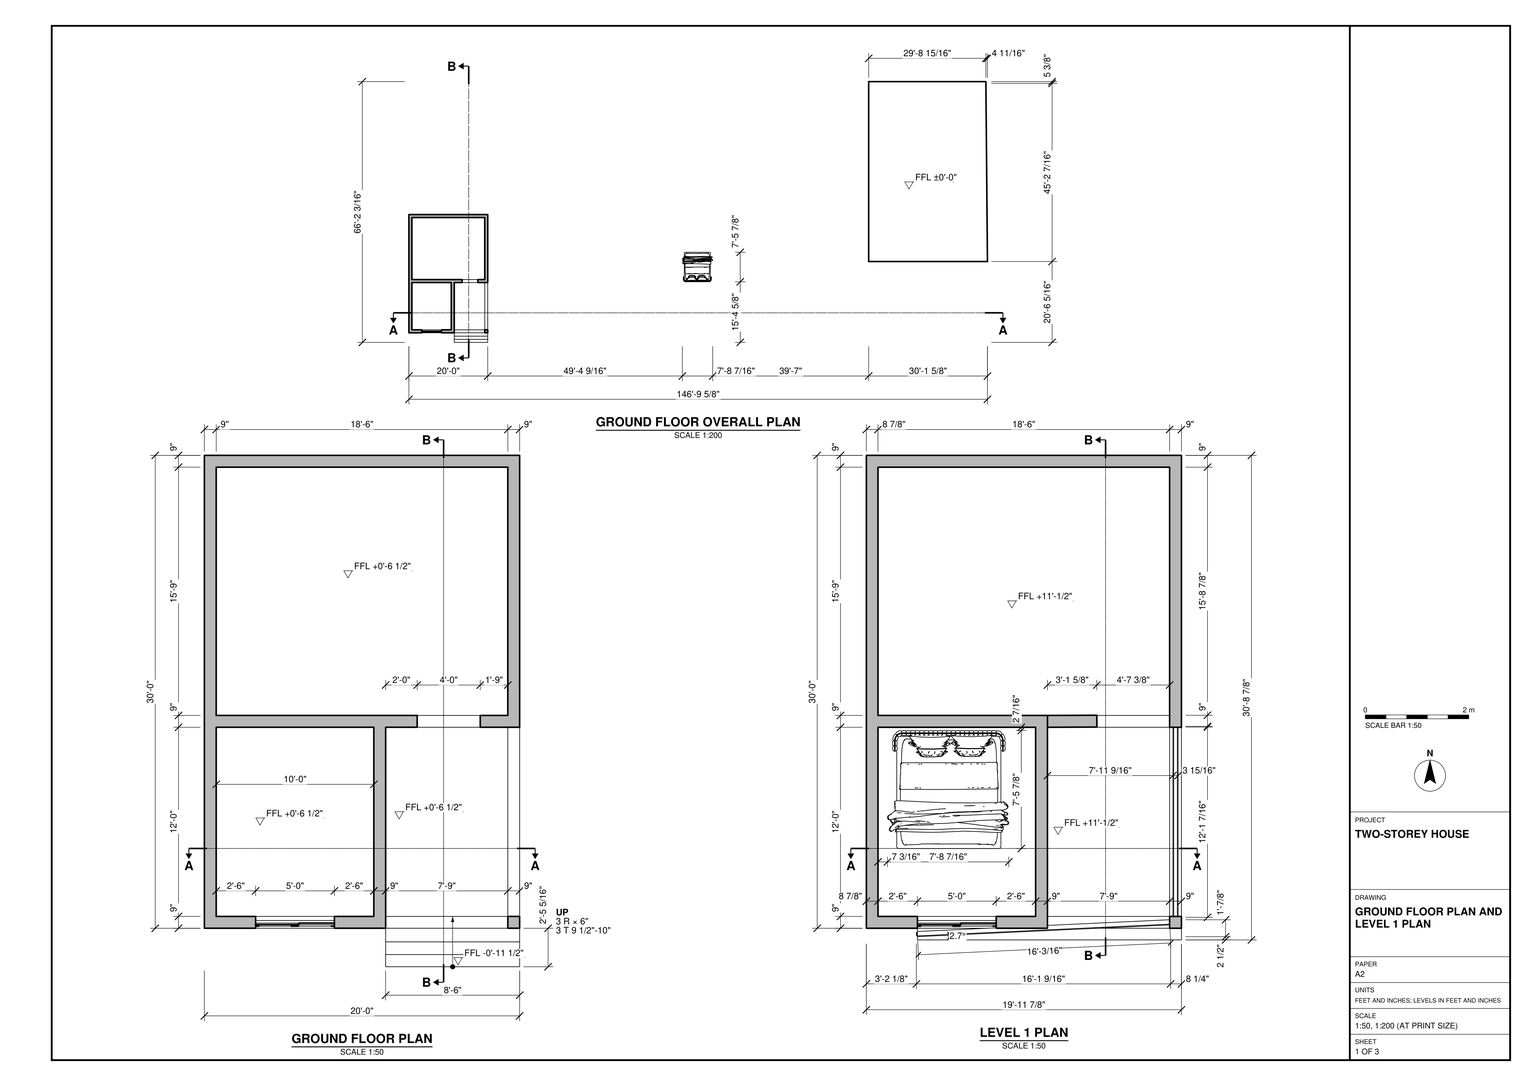
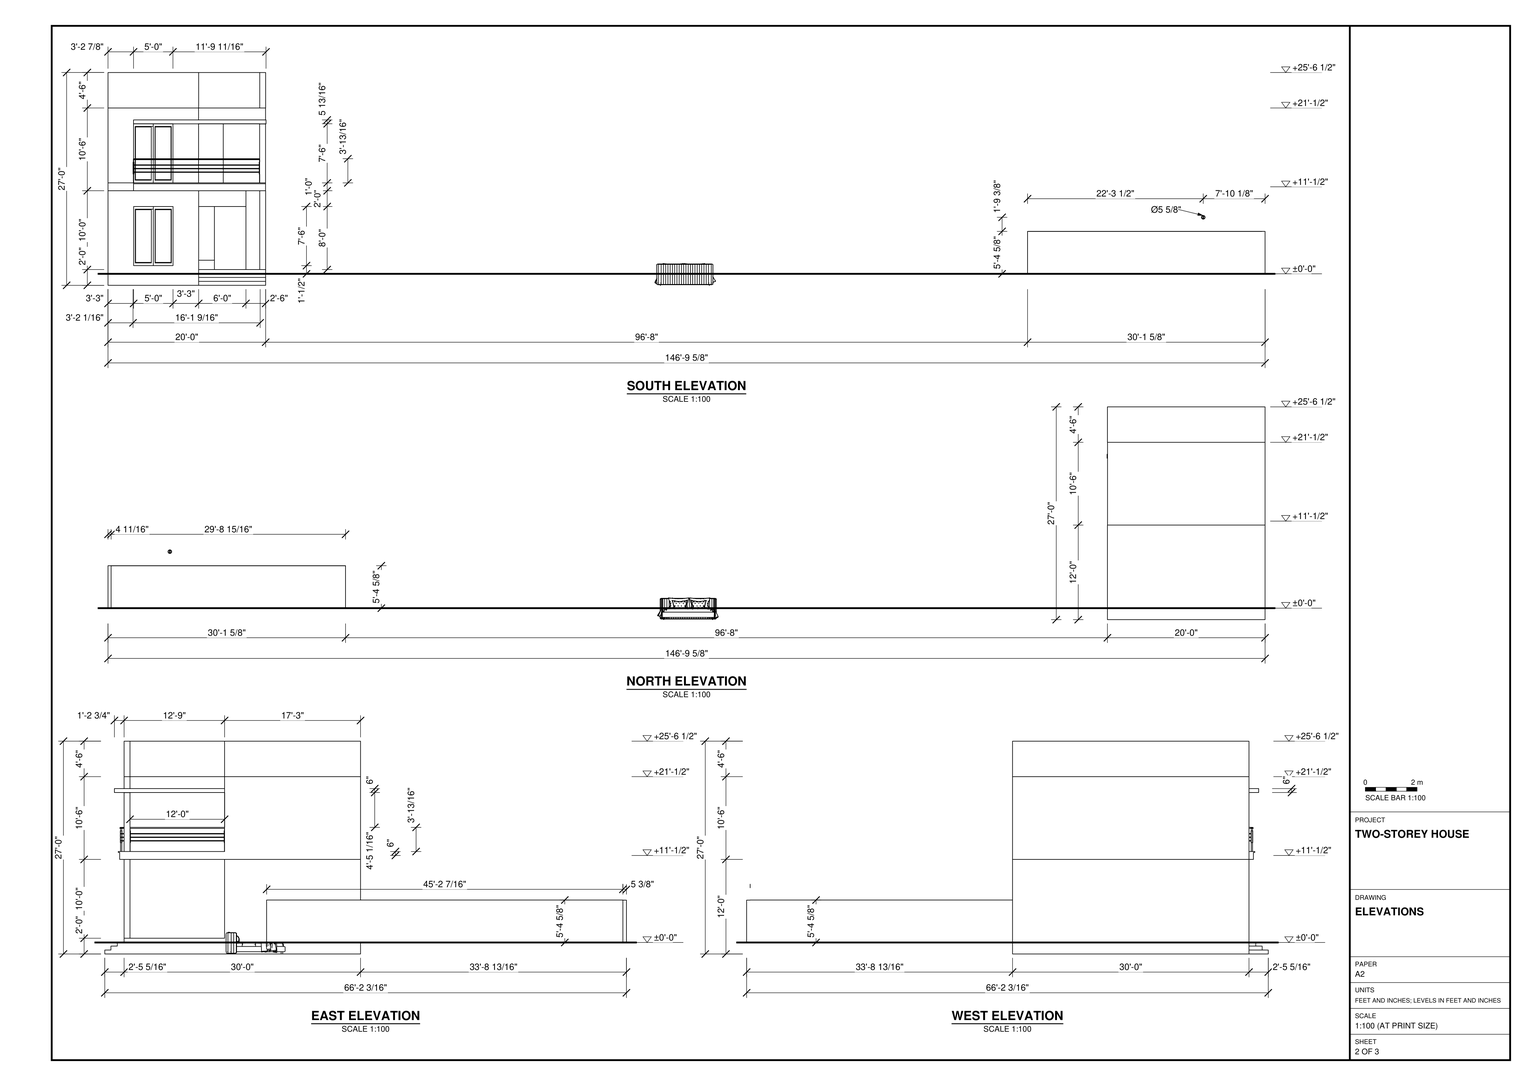
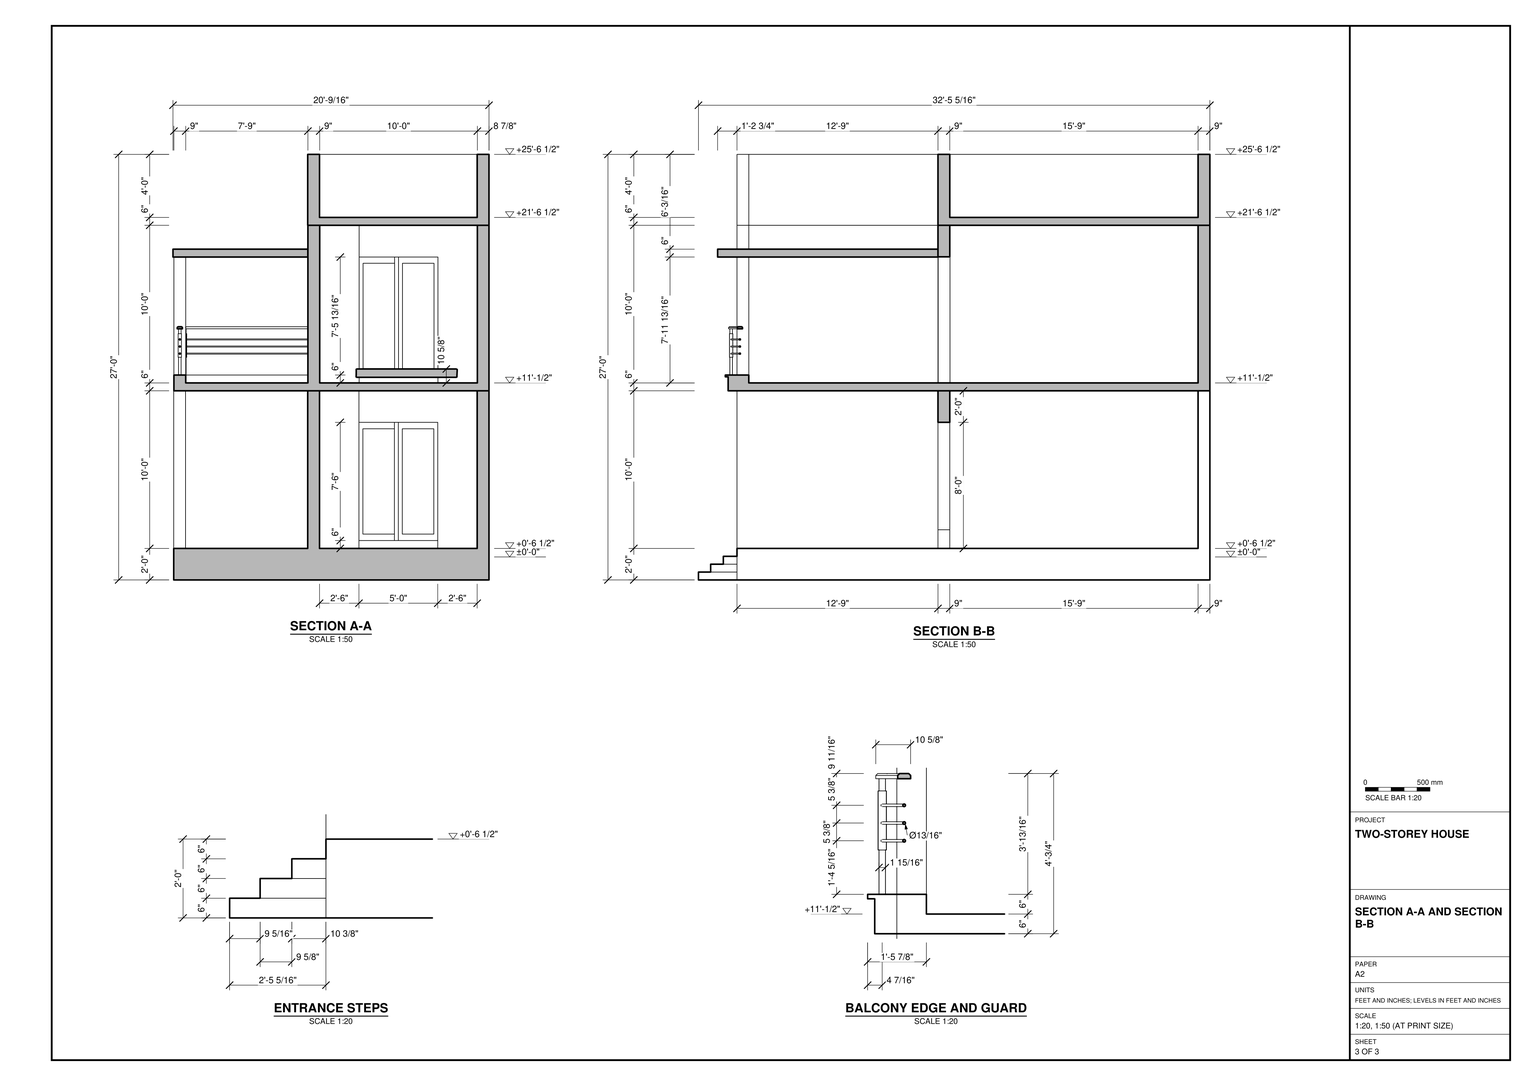
Build the house and the separate elements shown in task_files/diagram_01.pdf. Work in feet and inches. Use the overall plan to set out the full model: it measures 146'-9 5/8" east to west, 66'-2 3/16" north to south and 27'-0" high. Use ±0'-0" as the ground datum and +11'-1/2" as the upper floor level. The finished ground floor of the house sits above the datum at +0'-6 1/2".

Set out the 20'-0" by 30'-0" house at the west end. On each floor, form the full-width rear room and the smaller enclosed room at the front left, using the wall thicknesses shown in plan. Model the raised base, entrance steps, recessed entry bay, wall openings and framed window units. Follow the sections for the floor slabs, flat roof, parapets and lower canopy over the balcony. Include the balcony edge and horizontal guard rails. Place the bed in the upper front-left room as drawn. Use the overall plan and elevations to position the separate bed and the low rectangular element east of the house; they are not part of the house footprint.

Keep walls, slabs, roof elements and each furniture or joinery piece in separate groups or components, and use components for repeated parts. Decor and loose items may be any suitable library components. Save one SketchUp model as output_files/two_storey_house_with_a_covered_balcony.skp.

# SketchUp Ruby script. Lengths in inches.
U = 1.inch
M = Sketchup.active_model
def pt(a) = Geom::Point3d.new(a.map { |v| v * U })
def face(e, loops, mat)
  f = e.add_face(loops[0].map { |a| pt(a) })
  loops[1..].each { |l| e.add_face(l.map { |a| pt(a) }).erase! }
  f.material = f.back_material = mat if mat
  f
end
# faces: each face lists its corners as indices into pts; further lists are holes
def faces(e, pts, list, mat = nil) = list.each { |f| face(e, (f[0].is_a?(Array) ? f : [f]).map { |l| l.map { |i| pts[i] } }, mat) }
# xy, xz, yz: faces in a plane at the given z, y or x. An outline is a flat list of corners, or four numbers for a rectangle; further outlines are holes
def ring(l) = l.size == 4 ? [[l[0], l[1]], [l[2], l[1]], [l[2], l[3]], [l[0], l[3]]] : l.each_slice(2).to_a
def flat(e, list, mat, &to3) = list.each { |f| face(e, (f[0].is_a?(Array) ? f : [f]).map { |l| ring(l).map { |u, v| to3.(u, v) } }, mat) }
def xy(e, z, list, mat = nil) = flat(e, list, mat) { |x, y| [x, y, z] }
def xz(e, y, list, mat = nil) = flat(e, list, mat) { |x, z| [x, y, z] }
def yz(e, x, list, mat = nil) = flat(e, list, mat) { |y, z| [x, y, z] }
def lines(e, pts, list) = list.each { |a, b| e.add_line(pt(pts[a]), pt(pts[b])) }
# prism: a flat outline (further loops are holes) pulled along v
def prism(e, loops, v, mat = nil)
  f = face(e, loops, mat); d = Geom::Vector3d.new(v.map { |x| x * U })
  f.pushpull(f.normal.samedirection?(d) ? d.length : -d.length)
end
def box(e, o, s, mat = nil) = prism(e, [[o, [o[0] + s[0], o[1], o[2]], [o[0] + s[0], o[1] + s[1], o[2]], [o[0], o[1] + s[1], o[2]]]], [0, 0, s[2]], mat)
def at(x, y, z, deg = 0) = Geom::Transformation.translation(pt([x, y, z])) * Geom::Transformation.rotation(ORIGIN, Z_AXIS, deg.degrees)
def axes(o, x, y, z) = Geom::Transformation.new([*x, 0, *y, 0, *z, 0, *pt(o).to_a, 1])
def part(name) = M.definitions.add(name)
# library, detail: a bought-in or finely detailed component or shape, given as its bounding box
def library(name, o, s) = part(name).tap { |d| box(d.entities, o, s) }
def detail(e, o, s) = box(e.add_group.entities, o, s)
def put(e, d, t, mat = nil) = e.add_instance(d, t).tap { |i| i.material = mat if mat }
def group(e, t, mat = nil) = e.add_group.tap { |g| g.transformation = t; g.material = mat if mat }.entities
root = M.entities
M.materials.add("[Brick Antique 01]").color = [147, 105, 71]
M.materials.add("[Carrera Marble]").color = [207, 207, 207]
M.materials.add("[Color M05]").color = [114, 114, 114]
M.materials.add("[Color M08]").color = [30, 30, 30]
M.materials.add("[Color M09]").color = [0, 0, 0]
M.materials.add("[Translucent Glass Blue]").color = [100, 149, 237]
M.materials["[Translucent Glass Blue]"].alpha = 0.5
M.materials.add("[Wood Veneer 02]").color = [190, 128, 91]
c1 = part("Janela aluminio")
xy(c1.entities,0,[[0,0,47.24,1.57],[23.62,1.57,47.24,2.76],[0,2.76,25.98,3.9375],[0,3.9375,47.24,5.91]])
xy(c1.entities,43.31,[[0,0,47.24,1.57],[23.62,1.57,47.24,2.76],[0,2.76,0,5.91,47.24,5.91,47.24,3.9375,25.98,3.9375,25.98,2.76],[25.98,2.76,47.24,3.9375]])
xz(c1.entities,1.57,[[0,0,23.62,0,23.62,41.34,21.26,41.34,21.26,1.97,1.97,1.97,1.97,41.34,23.62,41.34,23.62,43.31,0,43.31],[[23.62,0,47.24,43.31],[25.7,1.97,45.28,41.34]]])
xz(c1.entities,2.76,[[[0,0,23.62,43.31],[2.36,2.36,21.26,40.94]],[23.62,0,25.98,43.31]])
xz(c1.entities,2.76,[[2.36,2.36,21.26,40.94]],"[Translucent Glass Blue]")
xz(c1.entities,3.9375,[[25.98,0,25.98,2.36,44.88,2.36,44.88,40.94,25.98,40.94,25.98,43.31,47.24,43.31,47.24,0]])
xz(c1.entities,3.9375,[[25.98,2.36,44.88,40.94]],"[Translucent Glass Blue]")
yz(c1.entities,0,[[0,0,1.57,43.31],[2.76,0,5.91,43.31]])
yz(c1.entities,23.62,[[1.57,0,2.76,43.31]])
yz(c1.entities,25.98,[[2.76,0,3.9375,43.31]])
yz(c1.entities,47.24,[[0,0,1.57,43.31],[1.57,0,2.76,43.31],[3.9375,0,5.91,43.31]])
c2 = library("Untitled",[0,-1.15,0],[92.42,91.04,33.3])
c3 = part("Ploe")
prism(c3.entities,[[[657.2,82.55,156],[657.29,80.58,156],[656.82,80.5625,156],[656.72,82.53,156]]],[0,0,36])
prism(c3.entities,[[[656.71,82.8,169.5],[656.83,80.29,169.5],[656.36,80.26,169.5],[656.24,82.78,169.5]]],[0,0,18],"[Wood Veneer 02]")
prism(c3.entities,[[[657.3,80.31,169.5],[657.18,82.83,169.5],[657.66,82.85,169.5],[657.77,80.33,169.5]]],[0,0,18],"[Wood Veneer 02]")
c4 = part("Group52\#1")
put(c4.entities,c3,at(0,0,0))
put(c4.entities,c3,at(1122.01,154.17,0,-180))
c5 = part("Ploe\#1")
box(c5.entities,[660.52,85.82,156],[1.97,0.47,36])
box(c5.entities,[660.25,86.29,169.5],[2.52,0.47,18],"[Wood Veneer 02]")
box(c5.entities,[660.25,85.35,169.5],[2.52,0.47,18],"[Wood Veneer 02]")
c6 = part("Group56\#1")
put(c6.entities,c5,at(0,0,0))
put(c6.entities,c5,at(1323.01,316.11,0,-180))
box(root,[231,29.33,24],[9,9,120])
p = [[39,38.33,24],[39,29.33,24],[99,38.33,24],[99,29.33,24],[162,182.33,24],[162,191.33,24],
  [210,182.33,24],[210,191.33,24]]
lines(root,p,[[0,1],[2,3],[4,5],[6,7]])
g1 = group(root,at(0,29.33,0))
box(g1,[230.86,0,156],[9,9,89.6875],"[Color M09]")
xy(g1,0,[[138,-29.33,138,0,0,0,0,360,240,360,240,-29.33]])
xy(g1,6,[[138,-29.33,240,-20.04]])
xy(g1,12,[[138,-20.04,240,-10.39]])
xy(g1,17.51,[[1400,217,1761.62,217,1756.91,759.46,1756.91,764.84,1400,764.84]])
xy(g1,18,[[138,-10.39,240,0]],"[Carrera Marble]")
xy(g1,24,[[9,9,129,153]])
xy(g1,24,[[138,0,231,9],[231,0,240,153],[138,9,231,153],[162,153,210,162],[9,162,231,351]],"[Carrera Marble]")
xy(g1,30,[[39,0,99,9]])
xy(g1,82.01,[[1400,759.46,1756.91,764.84]])
xy(g1,120,[[39,0,99,9],[162,153,210,162]])
xy(g1,144,[[0,0,138,0,138,153,210,153,210,162,9,162,9,153,129,153,129,9,9,9,9,351,231,351,231,153,240,153,240,360,0,360],[210,153,231,162]])
xy(g1,150,[[137.89,153,137.86,162,175.45,162.16,175.49,153.16]])
xy(g1,245.83,[[137.89,153,175.49,153.16,175.45,162.16,137.86,162]])
xy(g1,245.83,[[38.86,-14.75,38.86,0,137.89,0,137.89,153,240.5625,153,240.5625,-14.75]],"[Carrera Marble]")
xy(g1,251.83,[[38.86,-14.75,240.5625,-14.75,240.5625,153,137.89,153,137.89,0,38.86,0]],"[Carrera Marble]")
xy(g1,270,[[0,0,0,360,240,360,240,153,138,153,138,0]],"[Brick Antique 01]")
xy(g1,276,[[9,9,129,9,129,162,231,162,231,351,9,351]],"[Brick Antique 01]")
xy(g1,324,[[[0,0,138,0,138,153,240,153,240,360,0,360],[9,9,9,351,231,351,231,162,129,162,129,9]]],"[Brick Antique 01]")
xz(g1,-29.33,[[138,0,240,6]],"[Carrera Marble]")
xz(g1,-20.04,[[138,6,240,12]],"[Carrera Marble]")
xz(g1,-14.75,[[38.86,245.83,240.5625,251.83]],"[Carrera Marble]")
xz(g1,-10.39,[[138,12,240,18]],"[Carrera Marble]")
xz(g1,0,[[38.86,245.83,137.89,251.83]])
xz(g1,0,[[[0,0,138,144],[39,30,99,120]],[0,270,138,324]],"[Brick Antique 01]")
xz(g1,0,[[138,18,240,24],[231,24,240,144]],"[Carrera Marble]")
xz(g1,9,[[9,24,9,144,99,144,99,120,39,120,39,24],[39,24,99,30],[99,24,129,144]])
xz(g1,9,[[9,276,129,324]],"[Brick Antique 01]")
xz(g1,153,[[9,24,129,144],[137.89,245.83,240.5625,251.83]])
xz(g1,153,[[138,24,162,38.2],[210,24,231,144],[231,24,240,144],[138,38.2,162,120],[138,120,210,144],
  [138,270,231,324],[231,270,240,324]],"[Brick Antique 01]")
xz(g1,162,[[9,24,9,144,210,144,210,120,162,120,162,38.2,138,38.2,138,24],[138,24,162,38.2],[210,24,231,144]])
xz(g1,162,[[129,276,231,324]],"[Brick Antique 01]")
xz(g1,217,[[1400,17.51,1761.62,82.15]])
xz(g1,351,[[9,276,231,324]],"[Brick Antique 01]")
xz(g1,351,[[9,24,231,144]],"[Carrera Marble]")
xz(g1,360,[[0,0,240,144]])
xz(g1,360,[[0,270,240,324]],"[Brick Antique 01]")
xz(g1,759.46,[[1667.49,100.73,1667.58,100.74,1667.49,103.54,1667.39,100.74],[[1667.39,100.74,1667.49,103.54,1667.39,106.33,1666.76,106.25,1666.08,105.97,1665.5,105.52,1665.05,104.94,1664.77,104.26,1664.68,103.54,1664.77,102.81,1665.05,102.13,1665.5,101.55,1666.08,101.1,1666.76,100.82],[1666.96,101.24,1666.88,101.26,1666.31,101.49,1665.82,101.87,1665.44,102.36,1665.21,102.93,1665.13,103.54,1665.21,104.15,1665.44,104.72,1665.82,105.21,1666.31,105.58,1666.88,105.82,1666.96,105.83,1667.04,103.54]],[[1667.58,100.74,1668.22,100.82,1668.89,101.1,1669.48,101.55,1669.92,102.13,1670.2,102.81,1670.3,103.54,1670.2,104.26,1669.92,104.94,1669.48,105.52,1668.89,105.97,1668.22,106.25,1667.58,106.33,1667.49,103.54],[1668,101.23,1667.92,103.54,1668,105.84,1668.1,105.83,1668.67,105.59,1669.17,105.21,1669.54,104.72,1669.78,104.15,1669.86,103.54,1669.78,102.92,1669.54,102.35,1669.17,101.86,1668.67,101.48,1668.1,101.24]],[1668,101.23,1668.1,101.24,1668.67,101.48,1669.17,101.86,1669.54,102.35,1669.78,102.92,1669.86,103.54,1669.78,104.15,1669.54,104.72,1669.17,105.21,1668.67,105.59,1668.1,105.83,1668,105.84,1667.92,103.54],[1666.96,101.24,1667.04,103.54,1666.96,105.83,1666.88,105.82,1666.31,105.58,1665.82,105.21,1665.44,104.72,1665.21,104.15,1665.13,103.54,1665.21,102.93,1665.44,102.36,1665.82,101.87,1666.31,101.49,1666.88,101.26],
  [1667.49,103.54,1667.58,106.33,1667.49,106.35,1667.39,106.33]])
xz(g1,764.84,[[1400,17.51,1756.91,82.01]])
yz(g1,0,[[0,0,360,144],[0,270,360,324]],"[Brick Antique 01]")
yz(g1,9,[[9,24,153,144],[162,24,351,144]])
yz(g1,9,[[9,276,351,324]],"[Brick Antique 01]")
yz(g1,38.86,[[-14.75,245.83,0,251.83]])
yz(g1,39,[[0,30,9,120]])
yz(g1,99,[[0,30,9,120]])
yz(g1,129,[[9,24,153,144]])
yz(g1,129,[[9,276,162,324]],"[Brick Antique 01]")
yz(g1,137.89,[[0,245.83,153,251.83]])
yz(g1,138,[[0,24,153,144],[0,270,9,324],[9,270,153,324]],"[Brick Antique 01]")
yz(g1,138,[[-29.33,0,0,6],[-20.04,6,0,12],[-10.39,12,0,18]],"[Carrera Marble]")
yz(g1,162,[[153,24,162,38.2],[153,38.2,162,120]],"[Brick Antique 01]")
yz(g1,210,[[153,24,162,120]])
yz(g1,231,[[162,24,351,144]])
yz(g1,231,[[162,276,351,324]],"[Brick Antique 01]")
yz(g1,231,[[0,24,9,144]],"[Color M09]")
yz(g1,240,[[-29.33,0,360,0,360,144,153,144,153,24,0,24,0,18,-10.39,18,-10.39,12,-20.04,12,-20.04,6,-29.33,6],[153,270,360,324]],"[Brick Antique 01]")
yz(g1,240,[[0,24,9,144]],"[Color M08]")
yz(g1,240.5625,[[-14.75,245.83,153,251.83]],"[Carrera Marble]")
yz(g1,1400,[[217,17.51,764.84,17.51,764.84,82.01,759.46,82.01,759.46,82.15,217,82.15]])
yz(g1,1756.91,[[759.46,17.51,764.84,82.01]])
p = [[1761.62,217,17.51],[1761.62,217,82.15],[1756.91,759.46,82.15],[1756.91,759.46,82.01],[1756.91,759.46,17.51],[137.89,153,245.83],
  [137.86,162,245.83],[137.86,162,150],[137.89,153,150],[175.49,153.16,150],[175.49,153.16,245.83],[175.45,162.16,245.83],
  [175.45,162.16,150]]
faces(g1,p,[[0,1,2,3,4],[5,6,7,8],[7,6,11,12]])
faces(g1,p,[[5,8,9,10],[11,10,9,12]],"[Brick Antique 01]")
put(g1,c1,axes([39,0,30],[1.27,0,0],[0,1,0],[0,0,2.07818]),"[Color M09]")
put(g1,c1,axes([38.86,0,156],[1.27,0,0],[0,1,0],[0,0,2.07818]),"[Color M09]")
put(g1,c2,at(832.55,155.26,0))
put(g1,c2,at(108.48,150.54,150,180))
g2 = group(g1,at(0,-8.89,144),"[Brick Antique 01]")
xy(g2,0,[[38.86,2.16,38.86,8.89,0,8.89,0,368.89,239.86,368.89,239.86,2.16]])
xy(g2,6,[[8.86,17.89,128.86,161.89],[137.86,17.89,230.86,161.89],[137.86,161.89,230.86,170.89],[8.86,170.89,230.86,359.89]])
xy(g2,10.64,[[38.86,0,239.86,2.16]],"[Color M05]")
xy(g2,12,[[38.86,8.89,98.86,17.89],[137.86,8.89,239.86,8.89,239.86,161.89,230.86,161.89,230.86,17.89,137.86,17.89]])
xy(g2,12,[[38.86,0,239.86,8.89]],"[Color M05]")
xy(g2,101.83,[[38.86,8.89,98.86,17.89]])
xy(g2,102,[[137.86,161.89,230.86,170.89]])
xy(g2,126,[[[0,8.89,137.86,8.89,137.86,161.89,239.86,161.89,239.86,368.89,0,368.89],[8.86,170.89,230.86,359.89],[8.86,17.89,128.86,161.89]]])
xz(g2,0,[[38.86,10.64,239.86,12]],"[Color M05]")
xz(g2,2.16,[[38.86,0,239.86,10.64]],"[Color M05]")
xz(g2,8.89,[[0,0,38.86,12],[0,12,38.86,12,38.86,101.83,98.86,101.83,98.86,12,137.86,12,137.86,126,0,126]])
xz(g2,17.89,[[8.86,6,8.86,126,98.86,126,98.86,101.83,38.86,101.83,38.86,6],[38.86,6,98.86,12],[98.86,6,128.86,126],[137.86,6,230.86,12]])
xz(g2,161.89,[[8.86,6,128.86,126],[230.86,12,239.86,12,239.86,126,137.86,126,137.86,102,230.86,102]])
xz(g2,170.89,[[8.86,6,8.86,126,230.86,126,230.86,102,137.86,102,137.86,6]])
xz(g2,359.89,[[8.86,6,230.86,126]])
xz(g2,368.89,[[0,0,239.86,126]])
yz(g2,0,[[8.89,0,368.89,126]])
yz(g2,8.86,[[17.89,6,161.89,126],[170.89,6,359.89,126]])
yz(g2,38.86,[[8.89,12,17.89,101.83]])
yz(g2,38.86,[[2.16,0,2.16,10.64,0,10.64,0,12,8.89,12,8.89,0]],"[Color M05]")
yz(g2,98.86,[[8.89,12,17.89,101.83]])
yz(g2,128.86,[[17.89,6,161.89,126]])
yz(g2,137.86,[[17.89,6,161.89,126],[161.89,6,170.89,102],[8.89,12,17.89,126]])
yz(g2,230.86,[[17.89,6,161.89,12],[161.89,6,161.89,102,170.89,100.85,170.89,6],[170.89,6,359.89,126],[170.89,100.85,161.89,102,170.89,102]])
yz(g2,239.86,[[2.16,0,368.89,0,368.89,126,161.89,126,161.89,12,0,12,0,10.64,2.16,10.64]])
g3 = group(g1,at(38.09,-6.41,156))
g4 = group(g3,at(0.67,0,15.92))
prism(g4,[[[192.11,10.52,0.39],[192.11,10.53,0.29],[192.11,10.57,0.2],[192.1,10.63,0.12],[192.1,10.72,0.05],[192.1,10.81,0.01],[192.09,10.91,0],[192.09,11.01,0.01],[192.08,11.11,0.05],[192.08,11.19,0.12],[192.08,11.25,0.2],[192.07,11.29,0.29],[192.07,11.31,0.39],[192.07,11.29,0.5],[192.08,11.25,0.59],[192.08,11.19,0.67],[192.08,11.11,0.73],[192.09,11.01,0.77],[192.09,10.91,0.79],[192.1,10.81,0.77],[192.1,10.72,0.73],[192.1,10.63,0.67],[192.11,10.57,0.59],[192.11,10.53,0.5]]],[-192,-8.95,0])
prism(g4,[[[192.11,10.52,5.79],[192.11,10.53,5.69],[192.11,10.57,5.6],[192.1,10.63,5.52],[192.1,10.72,5.45],[192.1,10.81,5.41],[192.09,10.91,5.4],[192.09,11.01,5.41],[192.08,11.11,5.45],[192.08,11.19,5.52],[192.08,11.25,5.6],[192.07,11.29,5.69],[192.07,11.31,5.79],[192.07,11.29,5.9],[192.08,11.25,5.99],[192.08,11.19,6.07],[192.08,11.11,6.13],[192.09,11.01,6.17],[192.09,10.91,6.1875],[192.1,10.81,6.17],[192.1,10.72,6.13],[192.1,10.63,6.07],[192.11,10.57,5.99],[192.11,10.53,5.9]]],[-192,-8.95,0])
prism(g4,[[[192.11,10.52,11.19],[192.11,10.53,11.09],[192.11,10.57,11],[192.1,10.63,10.92],[192.1,10.72,10.85],[192.1,10.81,10.8125],[192.09,10.91,10.8],[192.09,11.01,10.8125],[192.08,11.11,10.85],[192.08,11.19,10.92],[192.08,11.25,11],[192.07,11.29,11.09],[192.07,11.31,11.19],[192.07,11.29,11.3],[192.08,11.25,11.39],[192.08,11.19,11.47],[192.08,11.11,11.53],[192.09,11.01,11.57],[192.09,10.91,11.59],[192.1,10.81,11.57],[192.1,10.72,11.53],[192.1,10.63,11.47],[192.11,10.57,11.39],[192.11,10.53,11.3]]],[-192,-8.95,0])
xy(g4,19.29,[[0.18,0,192,12.88,0,3.93],[0.18,0,192.18,8.95,192,12.88]],"[Wood Veneer 02]")
xy(g4,20.87,[[0.16,0.59,0.03,3.34,192.16,9.54],[0.03,3.34,192.03,12.29,192.16,9.54]],"[Wood Veneer 02]")
p = [[0,3.93,19.29],[0,3.93,20.28],[0.03,3.34,20.87],[0.16,0.59,20.87],[0.18,0,20.28],[0.18,0,19.29],
  [192.18,8.95,20.28],[192.18,8.95,19.29],[192,12.88,19.29],[192,12.88,20.28],[192.16,9.54,20.87],[192.03,12.29,20.87]]
faces(g4,p,[[0,1,2,3,4,5],[6,7,4],[4,7,5],[8,9,0],[0,9,1],[9,8,7,6,10,11],[3,6,4],[10,6,3],
  [1,11,2],[9,11,1]],"[Wood Veneer 02]")
put(g3,c4,at(-464.24,-70.64,-156))
g5 = group(g1,at(233.39,8.29,156))
put(g5,c6,at(-659.54,-85.35,-156))
g6 = group(g5,at(0,0.71,15.92))
prism(g6,[[[1.57,0,0.39],[1.59,0,0.29],[1.63,0,0.2],[1.69,0,0.12],[1.77,0,0.05],[1.87,0,0.01],[1.97,0,0],[2.07,0,0.01],[2.17,0,0.05],[2.25,0,0.12],[2.31,0,0.2],[2.35,0,0.29],[2.36,0,0.39],[2.35,0,0.5],[2.31,0,0.59],[2.25,0,0.67],[2.17,0,0.73],[2.07,0,0.77],[1.97,0,0.79],[1.87,0,0.77],[1.77,0,0.73],[1.69,0,0.67],[1.63,0,0.59],[1.59,0,0.5]]],[0,144,0])
prism(g6,[[[1.57,0,5.79],[1.59,0,5.69],[1.63,0,5.6],[1.69,0,5.52],[1.77,0,5.45],[1.87,0,5.41],[1.97,0,5.4],[2.07,0,5.41],[2.17,0,5.45],[2.25,0,5.52],[2.31,0,5.6],[2.35,0,5.69],[2.36,0,5.79],[2.35,0,5.9],[2.31,0,5.99],[2.25,0,6.07],[2.17,0,6.13],[2.07,0,6.17],[1.97,0,6.1875],[1.87,0,6.17],[1.77,0,6.13],[1.69,0,6.07],[1.63,0,5.99],[1.59,0,5.9]]],[0,144,0])
prism(g6,[[[1.57,0,11.19],[1.59,0,11.09],[1.63,0,11],[1.69,0,10.92],[1.77,0,10.85],[1.87,0,10.8125],[1.97,0,10.8],[2.07,0,10.8125],[2.17,0,10.85],[2.25,0,10.92],[2.31,0,11],[2.35,0,11.09],[2.36,0,11.19],[2.35,0,11.3],[2.31,0,11.39],[2.25,0,11.47],[2.17,0,11.53],[2.07,0,11.57],[1.97,0,11.59],[1.87,0,11.57],[1.77,0,11.53],[1.69,0,11.47],[1.63,0,11.39],[1.59,0,11.3]]],[0,144,0])
xy(g6,19.29,[[0,0,3.9375,0,0,144],[3.9375,0,3.9375,144,0,144]],"[Wood Veneer 02]")
xy(g6,20.87,[[0.59,0,0.59,144,3.35,144],[0.59,0,3.35,144,3.35,0]],"[Wood Veneer 02]")
xz(g6,0,[[0,19.29,0,20.28,0.59,20.87,3.35,20.87,3.9375,20.28,3.9375,19.29]],"[Wood Veneer 02]")
xz(g6,144,[[0,19.29,3.9375,19.29,3.9375,20.28,3.35,20.87,0.59,20.87,0,20.28]],"[Wood Veneer 02]")
yz(g6,0,[[0,19.29,144,19.29,144,20.28],[0,19.29,144,20.28,0,20.28]],"[Wood Veneer 02]")
yz(g6,3.9375,[[0,19.29,0,20.28,144,19.29],[144,19.29,0,20.28,144,20.28]],"[Wood Veneer 02]")
p = [[0.59,0,20.87],[0,0,20.28],[0.59,144,20.87],[0,144,20.28],[3.9375,0,20.28],[3.35,0,20.87],
  [3.9375,144,20.28],[3.35,144,20.87]]
faces(g6,p,[[0,1,2],[2,1,3],[4,5,6],[6,5,7]],"[Wood Veneer 02]")
